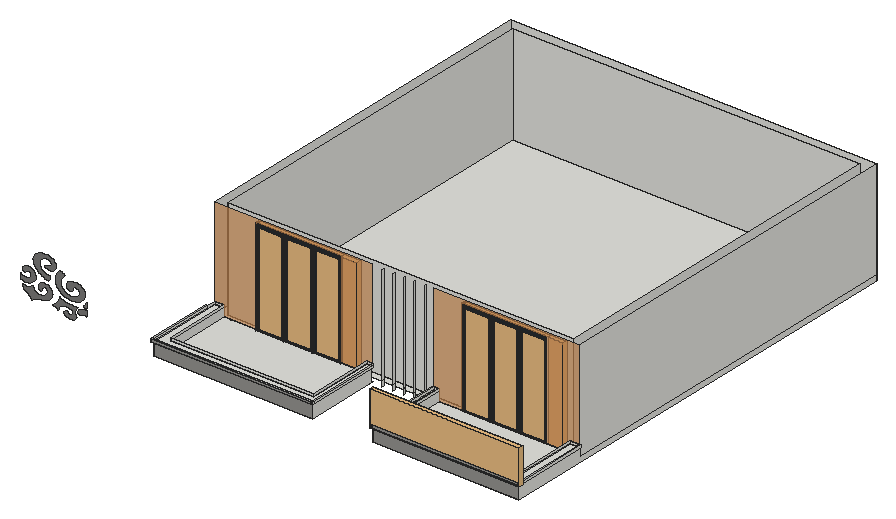
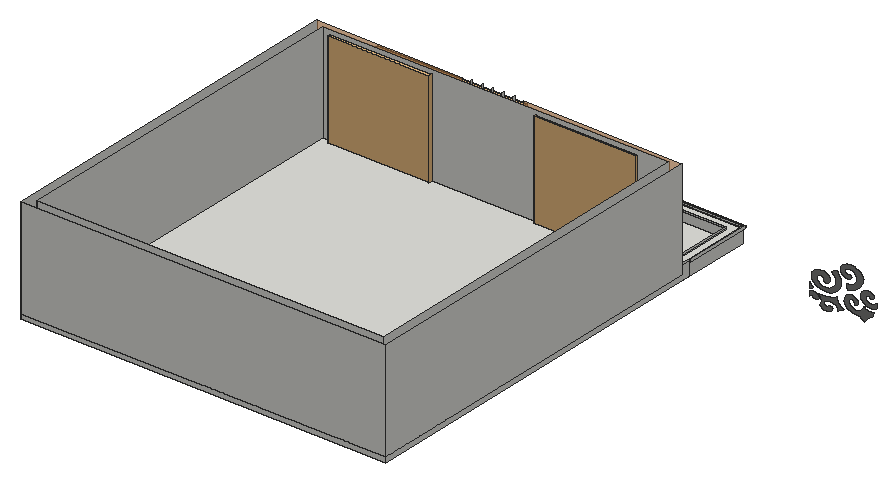
# SketchUp Ruby script. Lengths in inches.
U = 1.inch
M = Sketchup.active_model
def pt(a) = Geom::Point3d.new(a.map { |v| v * U })
def face(e, loops, mat)
  f = e.add_face(loops[0].map { |a| pt(a) })
  loops[1..].each { |l| e.add_face(l.map { |a| pt(a) }).erase! }
  f.material = f.back_material = mat if mat
  f
end
# faces: each face lists its corners as indices into pts; further lists are holes
def faces(e, pts, list, mat = nil) = list.each { |f| face(e, (f[0].is_a?(Array) ? f : [f]).map { |l| l.map { |i| pts[i] } }, mat) }
# xy, xz, yz: faces in a plane at the given z, y or x. An outline is a flat list of corners, or four numbers for a rectangle; further outlines are holes
def ring(l) = l.size == 4 ? [[l[0], l[1]], [l[2], l[1]], [l[2], l[3]], [l[0], l[3]]] : l.each_slice(2).to_a
def flat(e, list, mat, &to3) = list.each { |f| face(e, (f[0].is_a?(Array) ? f : [f]).map { |l| ring(l).map { |u, v| to3.(u, v) } }, mat) }
def xy(e, z, list, mat = nil) = flat(e, list, mat) { |x, y| [x, y, z] }
def xz(e, y, list, mat = nil) = flat(e, list, mat) { |x, z| [x, y, z] }
def yz(e, x, list, mat = nil) = flat(e, list, mat) { |y, z| [x, y, z] }
def lines(e, pts, list) = list.each { |a, b| e.add_line(pt(pts[a]), pt(pts[b])) }
# prism: a flat outline (further loops are holes) pulled along v
def prism(e, loops, v, mat = nil)
  f = face(e, loops, mat); d = Geom::Vector3d.new(v.map { |x| x * U })
  f.pushpull(f.normal.samedirection?(d) ? d.length : -d.length)
end
def box(e, o, s, mat = nil) = prism(e, [[o, [o[0] + s[0], o[1], o[2]], [o[0] + s[0], o[1] + s[1], o[2]], [o[0], o[1] + s[1], o[2]]]], [0, 0, s[2]], mat)
def at(x, y, z, deg = 0) = Geom::Transformation.translation(pt([x, y, z])) * Geom::Transformation.rotation(ORIGIN, Z_AXIS, deg.degrees)
def axes(o, x, y, z) = Geom::Transformation.new([*x, 0, *y, 0, *z, 0, *pt(o).to_a, 1])
def part(name) = M.definitions.add(name)
# library, detail: a bought-in or finely detailed component or shape, given as its bounding box
def library(name, o, s) = part(name).tap { |d| box(d.entities, o, s) }
def detail(e, o, s) = box(e.add_group.entities, o, s)
def put(e, d, t, mat = nil) = e.add_instance(d, t).tap { |i| i.material = mat if mat }
def group(e, t, mat = nil) = e.add_group.tap { |g| g.transformation = t; g.material = mat if mat }.entities
root = M.entities
M.materials.add("Wine2").color = [0, 0, 0]
M.materials["Wine2"].alpha = 0
M.materials.add("[0043_SaddleBrown]4").color = [124, 123, 122]
M.materials.add("[0130_Gainsboro]").color = [39, 45, 50]
M.materials.add("[Granite Light Gray]").color = [149, 148, 144]
M.materials.add("[Wood Floor Light]").color = [204, 176, 127]
M.materials.add("[Wood Floor]").color = [224, 152, 88]
M.materials["[Wood Floor]"].alpha = 0.68
c1 = part("Framed glazing panel")
xy(c1.entities,0,[[0,-0.98,43.07,0],[0,0,43.07,1.4]],"[0130_Gainsboro]")
xy(c1.entities,0.3,[[0.3,-1.43,42.77,-0.98]],"[0130_Gainsboro]")
xy(c1.entities,2.95,[[2.95,-1.43,40.12,-0.63],[2.95,-0.63,40.12,0],[2.95,0,40.12,0.64],[2.95,0.64,40.12,1.4]],"[0130_Gainsboro]")
xy(c1.entities,3.54,[[3.54,-0.63,39.53,0],[3.54,0,39.53,0.64]],"[0130_Gainsboro]")
xy(c1.entities,111.8125,[[3.54,-0.63,39.53,0],[3.54,0,39.53,0.64]],"[0130_Gainsboro]")
xy(c1.entities,112.4,[[2.95,-1.43,40.12,-0.63],[2.95,-0.63,40.12,0],[2.95,0,40.12,0.64],[2.95,0.64,40.12,1.4]],"[0130_Gainsboro]")
xy(c1.entities,115.05,[[0.3,-1.43,42.77,-0.98]],"[0130_Gainsboro]")
xy(c1.entities,115.35,[[0,-0.98,43.07,0],[0,0,43.07,1.4]],"[0130_Gainsboro]")
xz(c1.entities,-1.43,[[[0.3,0.3,42.77,115.05],[2.95,2.95,40.12,112.4]]],"[0130_Gainsboro]")
xz(c1.entities,-0.98,[[[0,0,43.07,115.35],[0.3,0.3,42.77,115.05]]],"[0130_Gainsboro]")
xz(c1.entities,-0.63,[[[2.95,2.95,40.12,112.4],[3.54,3.54,39.53,111.8125]]],"[0130_Gainsboro]")
xz(c1.entities,0,[[3.54,3.54,39.53,111.8125]],"Wine2")
xz(c1.entities,0,[[[0,0,43.07,115.35],[2.95,2.95,40.12,112.4]],[[2.95,2.95,40.12,112.4],[3.54,3.54,39.53,111.8125]]],"[0130_Gainsboro]")
xz(c1.entities,0.64,[[[2.95,2.95,40.12,112.4],[3.54,3.54,39.53,111.8125]]],"[0130_Gainsboro]")
xz(c1.entities,1.4,[[[0,0,43.07,115.35],[2.95,2.95,40.12,112.4]]],"[0130_Gainsboro]")
yz(c1.entities,0,[[-0.98,0,0,115.35],[0,0,1.4,115.35]],"[0130_Gainsboro]")
yz(c1.entities,0.3,[[-1.43,0.3,-0.98,115.05]],"[0130_Gainsboro]")
yz(c1.entities,2.95,[[-1.43,2.95,-0.63,112.4],[-0.63,2.95,0,112.4],[0,2.95,0.64,112.4],[0.64,2.95,1.4,112.4]],"[0130_Gainsboro]")
yz(c1.entities,3.54,[[-0.63,3.54,0,111.8125],[0,3.54,0.64,111.8125]],"[0130_Gainsboro]")
yz(c1.entities,39.53,[[-0.63,3.54,0,111.8125],[0,3.54,0.64,111.8125]],"[0130_Gainsboro]")
yz(c1.entities,40.12,[[-1.43,2.95,-0.63,112.4],[-0.63,2.95,0,112.4],[0,2.95,0.64,112.4],[0.64,2.95,1.4,112.4]],"[0130_Gainsboro]")
yz(c1.entities,42.77,[[-1.43,0.3,-0.98,115.05]],"[0130_Gainsboro]")
yz(c1.entities,43.07,[[-0.98,0,0,115.35],[0,0,1.4,115.35]],"[0130_Gainsboro]")
c2 = part("Glazing assembly")
put(c2.entities,c1,axes([90.57,1.43,0],[1.05148,0,0],[0,1,0],[0,0,1]))
put(c2.entities,c1,axes([0,1.43,0],[1.05148,0,0],[0,1,0],[0,0,1]))
put(c2.entities,c1,axes([45.29,1.43,0],[1.05148,0,0],[0,1,0],[0,0,1]))
c3 = library("Curtains",[0,0,0],[121.73,8.19,117.22])
c4 = library("Glass Railing",[0,0,0],[139.5,4.76,42])
xy(root,388.875,[[602.01,651.03,703.26,657.03],[849.76,651.03,951.01,657.03]])
xy(root,394.4375,[[551.76,559.875,742.44,570.83],[814.89,559.875,990.19,570.83],[563.08,657.03,978.86,1085.17]])
xy(root,394.4375,[[551.76,570.83,563.08,651.03],[563.08,570.83,742.44,651.03],[814.89,570.83,978.86,651.03],[978.86,570.83,990.19,651.03]],"[Wood Floor Light]")
xy(root,400.4375,[[563.08,570.83,734.59,570.83,734.59,651.03,703.26,651.03,703.26,657.03,602.01,657.03,602.01,651.03,563.08,651.03],[820.97,570.83,978.86,570.83,978.86,651.03,951.01,651.03,951.01,657.03,849.76,657.03,849.76,651.03,820.97,651.03],[551.76,651.03,551.76,1096.5,990.19,1096.5,990.19,651.03,951.01,651.03,951.01,657.03,978.86,657.03,978.86,1085.17,563.08,1085.17,563.08,657.03,602.01,657.03,602.01,651.03],[563.08,657.03,978.86,1085.17]])
xy(root,410.625,[[550.01,557.9375,742.44,559.875],[742.44,557.9375,744.38,559.875],[812.96,557.9375,814.89,559.875],[814.89,557.9375,990.19,559.875],[990.19,557.9375,992.12,559.875],
  [549.82,559.875,551.76,640.11],[551.76,559.875,551.76,651.03,563.08,651.03,563.08,570.83,734.59,570.83,734.59,651.03,742.44,651.03,742.44,559.875],[742.44,559.875,744.38,647.91],[812.96,559.875,814.89,651.03],[814.89,559.875,814.89,651.03,820.97,651.03,820.97,570.83,978.86,570.83,978.86,651.03,990.19,651.03,990.19,559.875],
  [990.19,559.875,992.12,651.03]])
xz(root,557.9375,[[990.19,410.625,992.12,413.5]])
xz(root,557.9375,[[550.01,410.625,742.44,413.5],[742.44,410.625,744.38,413.5],[812.96,410.625,814.89,413.5],[814.89,410.625,990.19,413.5]],"[Granite Light Gray]")
xz(root,559.875,[[549.82,410.625,550.01,413.5],[550.01,410.625,551.76,413.5],[551.76,410.625,742.44,413.5],[742.44,410.625,744.38,413.5],[812.96,410.625,814.89,413.5],
  [814.89,410.625,990.19,413.5],[990.19,410.625,992.12,413.5]])
xz(root,559.875,[[551.76,394.4375,742.44,410.625],[814.89,394.4375,990.19,410.625]],"[Granite Light Gray]")
xz(root,570.83,[[563.08,400.4375,734.59,410.625],[820.97,400.4375,978.86,410.625],[563.08,410.625,734.59,413.5],[820.97,410.625,978.86,413.5]])
xz(root,589.17,[[427.53,378.34,429.1875,378.37,430.81,378.64,432.3125,379.15,433.64,379.86,434.74,380.76,435.56,381.8,435,382.74,434.55,383.71,434.23,384.71,434.03,385.72,433.95,386.75,434,387.77,434.18,388.79,434.48,389.79,434.9,390.76,435.44,391.71,436.1,392.62,436.86,393.48,434.98,393.37,433.1,393.33,431.21,393.38,429.34,393.5,427.47,393.71,425.63,393.99,423.81,394.35,422.02,394.79,420.28,395.3,418.57,395.88,416.92,396.54,415.32,397.26,415.21,396.19,414.98,395.13,414.64,394.09,414.19,393.07,413.64,392.07,412.99,391.11,412.24,390.1875,411.39,389.31,410.46,388.47,409.4375,387.69,408.34,386.97,407.17,386.31,407.79,386.1,408.4,385.89,409.01,385.67,409.61,385.44,410.2,385.2,410.79,384.95,411.37,384.7,411.94,384.44,412.5,384.16,413.0625,383.88,413.61,383.59,414.15,383.3,414.26,384.7,414.78,386.05,415.7,387.29,416.98,388.35,418.54,389.19,420.32,389.77,422.22,390.05,424.17,390.03,426.07,389.7,427.82,389.08,429.34,388.2,430.56,387.11,430.6,386.77,430.62,386.43,430.62,385.75,430.56,385.07,430.51,384.73,430.44,384.39,430.36,384.06,430.27,383.72,430.17,383.39,430.04,383.06,429.45,382.875,428.82,382.76,428.18,382.72,427.53,382.75,426.9,382.85,426.3,383.03,425.75,383.27,425.25,383.58,424.83,383.93,424.5,384.33,424.25,384.76,424.11,385.22,423.7,385.09,423.3125,384.95,422.93,384.79,422.57,384.61,422.22,384.41,421.89,384.2,421.58,383.98,421.28,383.74,421.01,383.48,420.77,383.22,420.54,382.95,420.34,382.66,420.93,381.54,421.82,380.53,422.98,379.68,424.36,379.01,425.89,378.55],[381.96,382.25,382.57,383.03,383.29,383.77,384.1,384.44,385.01,385.06,386,385.6,387.0625,386.07,388.19,386.46,389.36,386.77,390.57,386.98,391.8,387.11,393.04,387.15,394.29,387.09,396.7,387.5,398.99,388.2,401.07,389.18,402.875,390.4,404.36,391.84,405.48,393.4375,406.19,395.15,406.48,396.93,406.33,398.71,405.76,400.46,404.77,402.1,403.4,403.59,402.27,404.41,400.93,405.05,399.43,405.47,397.84,405.65,396.24,405.59,394.6875,405.29,393.26,404.75,392.02,404.02,391.02,403.11,390.31,402.07,389.91,400.95,389.86,399.79,389.92,399.43,390.03,399.08,390.19,398.73,390.4,398.4,390.66,398.09,390.96,397.8,391.3,397.53,391.67,397.29,392.08,397.08,392.52,396.9,392.98,396.75,393.46,396.64,393.54,397.15,393.66,397.65,393.82,398.15,394.03,398.64,394.27,399.13,394.55,399.6,394.87,400.06,395.23,400.5,395.62,400.93,396.04,401.34,396.5,401.74,396.99,402.11,397.92,401.77,398.77,401.34,399.52,400.81,400.15,400.2,400.64,399.54,400.98,398.83,401.17,398.08,401.19,397.33,401.05,396.58,400.76,395.86,400.32,395.18,399.73,394.55,398.89,393.61,397.82,392.8,396.57,392.14,395.17,391.66,393.67,391.38,392.12,391.3,390.58,391.43,389.09,391.76,387.72,392.28,386.51,392.98,385.49,393.82,384.71,394.79,384.49,395.05,384.29,395.3125,384.1,395.58,383.92,395.85,383.75,396.13,383.6,396.41,383.46,396.69,383.33,396.98,383.22,397.27,383.11,397.5625,383.02,397.86,382.95,398.15,382.26,397.49,381.46,396.89,380.56,396.375,379.58,395.94,378.53,395.6,377.4375,395.35,376.3,395.2,375.16,395.16,374.01,395.22,372.88,395.38,371.79,395.64,370.75,396,370.97,395.6875,371.16,395.37,371.32,395.04,371.46,394.71,371.58,394.375,371.66,394.03,371.72,393.6875,371.75,393.34,371.76,392.99,371.73,392.65,371.68,392.3,371.6,391.96,372.75,391.33,373.84,390.67,374.9,389.96,375.9,389.22,376.86,388.45,377.76,387.64,378.61,386.81,379.4,385.95,380.13,385.06,380.8,384.14,381.41,383.2],[440.07,386.82,440.61,386.85,441.07,386.92,441.53,387.02,441.96,387.15,442.38,387.31,442.78,387.49,443.16,387.7,443.51,387.93,443.83,388.18,444.11,388.45,444.36,388.74,444.58,389.05,444.76,389.36,445.1,389.23,445.4375,389.09,445.77,388.93,446.09,388.77,446.41,388.6,446.72,388.43,447.02,388.24,447.31,388.05,447.59,387.85,447.86,387.65,448.12,387.4375,448.37,387.22,448.37,393,447.39,393.38,446.35,393.65,445.26,393.8,444.15,393.8125,443.05,393.7,441.99,393.47,440.99,393.11,440.09,392.65,439.3,392.09,438.64,391.45,438.13,390.73,437.79,389.97,437.53,389.63,437.375,389.25,437.32,388.86,437.37,388.47,437.53,388.09,437.78,387.74,438.12,387.4375,438.53,387.18,439.01,386.99,439.53,386.87],[447.98,396.46,448.37,396.47,448.37,402.56,448.09,402.125,447.79,401.6875,447.49,401.26,447.17,400.83,446.84,400.41,446.5,399.99,446.15,399.58,445.79,399.18,445.41,398.77,445.03,398.38,444.63,397.99,444.22,397.61,444.5,397.42,444.79,397.24,445.1,397.08,445.43,396.9375,445.77,396.8125,446.12,396.71,446.48,396.62,446.85,396.55,447.22,396.5,447.6,396.47],[429.86,398.78,432.06,398.88,434.23,399.21,436.31,399.74,438.27,400.47,440.07,401.39,441.69,402.47,443.08,403.7,444.23,405.0625,445.11,406.52,445.71,408.05,446.02,409.625,446.01,410.99,445.73,412.35,445.18,413.65,444.36,414.89,443.31,416.03,442.04,417.04,440.57,417.91,438.94,418.61,437.19,419.14,435.35,419.47,433.47,419.61,431.57,419.54,430.1,419.33,428.69,418.9375,427.4,418.39,426.24,417.7,425.26,416.875,424.48,415.95,423.92,414.95,423.59,413.89,423.51,412.81,423.68,411.73,424.09,410.68,424.73,409.7,425.24,409.31,425.86,409,426.55,408.79,427.29,408.68,428.04,408.6875,428.77,408.8,429.46,409.03,430.07,409.35,430.57,409.75,430.95,410.22,431.18,410.73,431.07,411.09,431.01,411.45,431.01,411.81,431.0625,412.17,431.17,412.52,431.34,412.87,431.55,413.19,431.82,413.5,432.13,413.79,432.48,414.04,432.875,414.27,433.3,414.46,434.31,414.36,435.29,414.15,436.21,413.83,437.05,413.41,437.79,412.9,438.41,412.32,438.91,411.68,439.26,410.98,439.46,410.26,439.5,409.53,439.39,408.8,439.12,408.08,438.37,406.9,437.36,405.82,436.11,404.88,434.67,404.1,433.0625,403.5,431.34,403.11,429.55,402.93,427.75,402.96,425.98,403.22,424.29,403.68,422.73,404.34,421.35,405.17,419.9,406.36,418.67,407.66,417.7,409.08,416.99,410.57,416.5625,412.12,416.42,413.7,416.5625,415.27,416.99,416.82,417.7,418.3125,418.67,419.73,419.9,421.04,421.35,422.22,420.98,422.57,420.6,422.9,420.19,423.22,419.77,423.53,419.33,423.82,418.86,424.1,418.38,424.37,417.89,424.61,417.38,424.84,416.85,425.06,416.32,425.25,415.77,425.43,414.64,424.36,413.63,423.23,412.74,422.04,411.98,420.8125,411.34,419.55,410.84,418.25,410.47,416.93,410.24,415.6,410.15,414.25,410.19,412.91,410.375,411.57,410.7,410.24,411.23,408.8125,411.96,407.43,412.88,406.1,413.98,404.85,415.26,403.69,416.69,402.63,418.26,401.68,419.97,400.85,421.77,400.15,423.67,399.58,425.64,399.16,427.66,398.88],
  [374.97,399.74,376.05,399.78,377.11,399.9,378.15,400.1,379.17,400.36,380.14,400.7,381.83,401.49,383.33,402.47,384.59,403.61,385.58,404.88,386.28,406.25,386.66,407.68,386.72,409.14,386.46,410.58,385.88,411.98,384.99,413.29,383.83,414.48,382.42,415.52,381.4375,416.12,380.32,416.58,379.1,416.875,377.83,417,376.55,416.95,375.3,416.72,374.13,416.33,373.09,415.79,372.21,415.12,371.52,414.34,371.04,413.48,370.8,412.57,370.71,412.22,370.72,411.86,370.82,411.51,371.01,411.18,371.29,410.89,371.65,410.63,372.06,410.4375,372.52,410.3,373,410.24,373.5,410.24,373.99,410.31,374.44,410.45,374.71,410.7,375,410.9375,375.31,411.17,375.64,411.38,375.98,411.58,376.35,411.76,376.72,411.92,377.12,412.07,377.52,412.2,377.93,412.31,378.36,412.4,378.78,412.47,379.35,412.12,379.85,411.73,380.28,411.29,380.625,410.82,380.9,410.32,381.08,409.8,381.17,409.27,381.17,408.74,381.08,408.2,380.9,407.69,380.64,407.1875,380.29,406.71,379.5625,406,378.68,405.39,377.66,404.89,376.54,404.53,375.36,404.3,374.13,404.23,372.91,404.3,371.72,404.53,370.6,404.89,369.59,405.39,368.7,406,367.98,406.71,367.98,401.47,368.85,401.01,369.78,400.625,370.76,400.3,371.78,400.05,372.83,399.875,373.9,399.77],[402,409.96,402.41,410.4,402.78,410.87,403.09,411.35,403.35,411.86,403.5625,412.37,403.72,412.89,403.82,413.42,403.86,413.96,403.85,414.49,403.79,415.03,403.67,415.56,403.49,416.08,402.14,415.96,400.78,415.98,399.44,416.14,398.13,416.43,396.9,416.85,395.76,417.38,394.73,418.02,393.83,418.76,393.09,419.58,392.51,420.47,392.1,421.4,391.875,422.37,391.51,423.29,391.28,424.22,391.1875,425.17,391.24,426.125,391.43,427.06,391.77,427.99,392.23,428.875,392.83,429.73,393.55,430.52,394.38,431.26,395.32,431.93,396.35,432.53,397.31,432.92,398.35,433.1875,399.45,433.3,400.55,433.26,401.625,433.08,402.63,432.75,403.54,432.29,404.3,431.71,404.9,431.04,405.32,430.3,405.53,429.52,405.53,428.72,405.45,428.33,405.29,427.95,405.06,427.59,404.76,427.25,404.4,426.95,403.99,426.6875,403.53,426.46,403.04,426.29,402.51,426.16,401.97,426.09,401.42,426.07,400.87,426.11,400.3,426.125,399.73,426.05,399.21,425.88,398.75,425.63,398.38,425.3125,398.12,424.94,397.99,424.54,397.98,424.13,398.11,423.72,398.36,423.35,398.72,423.03,399.17,422.77,400.41,422.33,401.75,422.0625,403.14,421.97,404.52,422.0625,405.86,422.33,407.1,422.77,408.22,423.37,409.16,424.1,409.91,424.95,410.43,425.875,410.71,426.86,410.73,427.86,410.79,429.07,410.61,430.28,410.21,431.45,409.58,432.58,408.75,433.63,407.73,434.59,406.53,435.44,405.18,436.17,403.7,436.75,402.13,437.18,400.49,437.46,398.82,437.5625,396.48,437.47,394.2,437.11,392.02,436.49,390,435.64,388.1875,434.58,386.63,433.32,385.36,431.9,384.42,430.36,383.82,428.73,383.58,427.05,383.71,425.37,384.2,423.72,384.75,422.12,385.51,420.56,386.46,419.06,387.6,417.63,388.91,416.28,390.4,415.02,392.03,413.87,393.81,412.83,395.71,411.91,397.72,411.12,399.82,410.47]],"[0043_SaddleBrown]4")
xz(root,640.11,[[549.82,410.625,551.76,413.5]])
xz(root,647.91,[[742.44,410.625,744.38,413.5]])
xz(root,651.03,[[551.76,400.4375,563.08,410.625],[978.86,400.4375,990.19,410.625],[551.76,410.625,563.08,413.5],[734.59,410.625,742.44,413.5],[812.96,410.625,814.68,413.5],
  [814.68,410.625,814.89,413.5],[814.89,410.625,820.97,413.5],[978.86,410.625,990.19,413.5],[990.19,410.625,992.12,413.5]])
xz(root,651.03,[[563.08,400.4375,602.01,400.4375,602.01,514.875,703.26,514.875,703.26,400.4375,734.59,400.4375,734.59,413.5,742.44,413.5,742.44,520.4375,551.76,520.4375,551.76,413.5,563.08,413.5],[820.97,400.4375,849.76,400.4375,849.76,514.875,951.01,514.875,951.01,400.4375,978.86,400.4375,978.86,413.5,990.19,413.5,990.19,520.4375,814.89,520.4375,814.89,413.5,820.97,413.5]],"[Wood Floor]")
xz(root,657.03,[[563.08,400.4375,563.08,520.4375,978.86,520.4375,978.86,400.4375,951.01,400.4375,951.01,514.875,849.76,514.875,849.76,400.4375,703.26,400.4375,703.26,514.875,602.01,514.875,602.01,400.4375]])
xz(root,1085.17,[[563.08,400.4375,978.86,520.4375]])
xz(root,1096.5,[[551.76,394.4375,990.19,400.4375],[551.76,400.4375,990.19,520.4375]])
yz(root,549.82,[[559.875,410.625,640.11,413.5]])
yz(root,550.01,[[557.9375,410.625,559.875,413.5]])
yz(root,551.76,[[559.875,394.4375,640.11,410.625],[640.11,394.4375,640.11,410.625,651.03,410.625,651.03,400.4375,1096.5,400.4375,1096.5,394.4375],[651.03,400.4375,1096.5,520.4375],[559.875,410.625,640.11,413.5],[640.11,410.625,651.03,413.5]])
yz(root,563.08,[[570.83,400.4375,651.03,410.625],[657.03,400.4375,1085.17,520.4375],[570.83,410.625,651.03,413.5]])
yz(root,602.01,[[651.03,400.4375,657.03,514.875]])
yz(root,703.26,[[651.03,400.4375,657.03,514.875]])
yz(root,734.59,[[570.83,400.4375,651.03,410.625],[570.83,410.625,651.03,413.5]])
yz(root,742.44,[[559.875,394.4375,647.91,410.625],[557.9375,410.625,559.875,413.5],[559.875,410.625,647.91,413.5],[647.91,410.625,651.03,413.5]])
yz(root,744.38,[[557.9375,410.625,559.875,413.5],[559.875,410.625,647.91,413.5]])
yz(root,755.44,[[647.91,394.4375,651.03,400.4375],[647.91,400.4375,651.03,520.4375]])
yz(root,768.19,[[648.85,394.4375,651.03,400.4375],[648.85,400.4375,651.03,520.4375]])
yz(root,780.32,[[648.85,394.4375,651.03,400.4375],[648.85,400.4375,651.03,520.4375]])
yz(root,792.69,[[648.85,394.4375,651.03,400.4375],[648.85,400.4375,651.03,520.4375]])
yz(root,805.57,[[648.85,394.4375,651.03,400.4375],[648.85,400.4375,651.03,520.4375]])
yz(root,812.96,[[557.9375,410.625,559.875,413.5],[559.875,410.625,651.03,413.5]])
yz(root,814.89,[[559.875,394.4375,651.03,410.625],[557.9375,410.625,559.875,413.5],[559.875,410.625,651.03,413.5]])
yz(root,820.97,[[570.83,400.4375,651.03,410.625],[570.83,410.625,651.03,413.5]])
yz(root,849.76,[[651.03,400.4375,657.03,514.875]])
yz(root,951.01,[[651.03,400.4375,657.03,514.875]])
yz(root,978.86,[[570.83,400.4375,651.03,410.625],[657.03,400.4375,1085.17,520.4375],[570.83,410.625,651.03,413.5]])
yz(root,990.19,[[559.875,394.4375,1096.5,394.4375,1096.5,400.4375,651.03,400.4375,651.03,410.625,559.875,410.625],[651.03,400.4375,1096.5,520.4375],[557.9375,410.625,559.875,413.5],[559.875,410.625,651.03,413.5]])
yz(root,992.12,[[557.9375,410.625,559.875,413.5],[559.875,410.625,651.03,413.5]])
p = [[431.27,589.17,411.27],[431.18,589.17,410.73]]
lines(root,p,[[0,1]])
put(root,c2,axes([601.61,650.7,397.79],[0.75,0,0],[0,0.75,0],[0,0,1.01765]))
put(root,c3,at(600.82,651.68,397.95))
put(root,c2,axes([849.11,651.03,397.48],[0.75,0,0],[0,0.75,0],[0,0,1.01765]))
put(root,c4,axes([812.96,558.12,409.93],[1.28434,0,0],[0,1,0],[0,0,1]),"[Granite Light Gray]")
put(root,c3,at(847.86,652.22,397.95))
